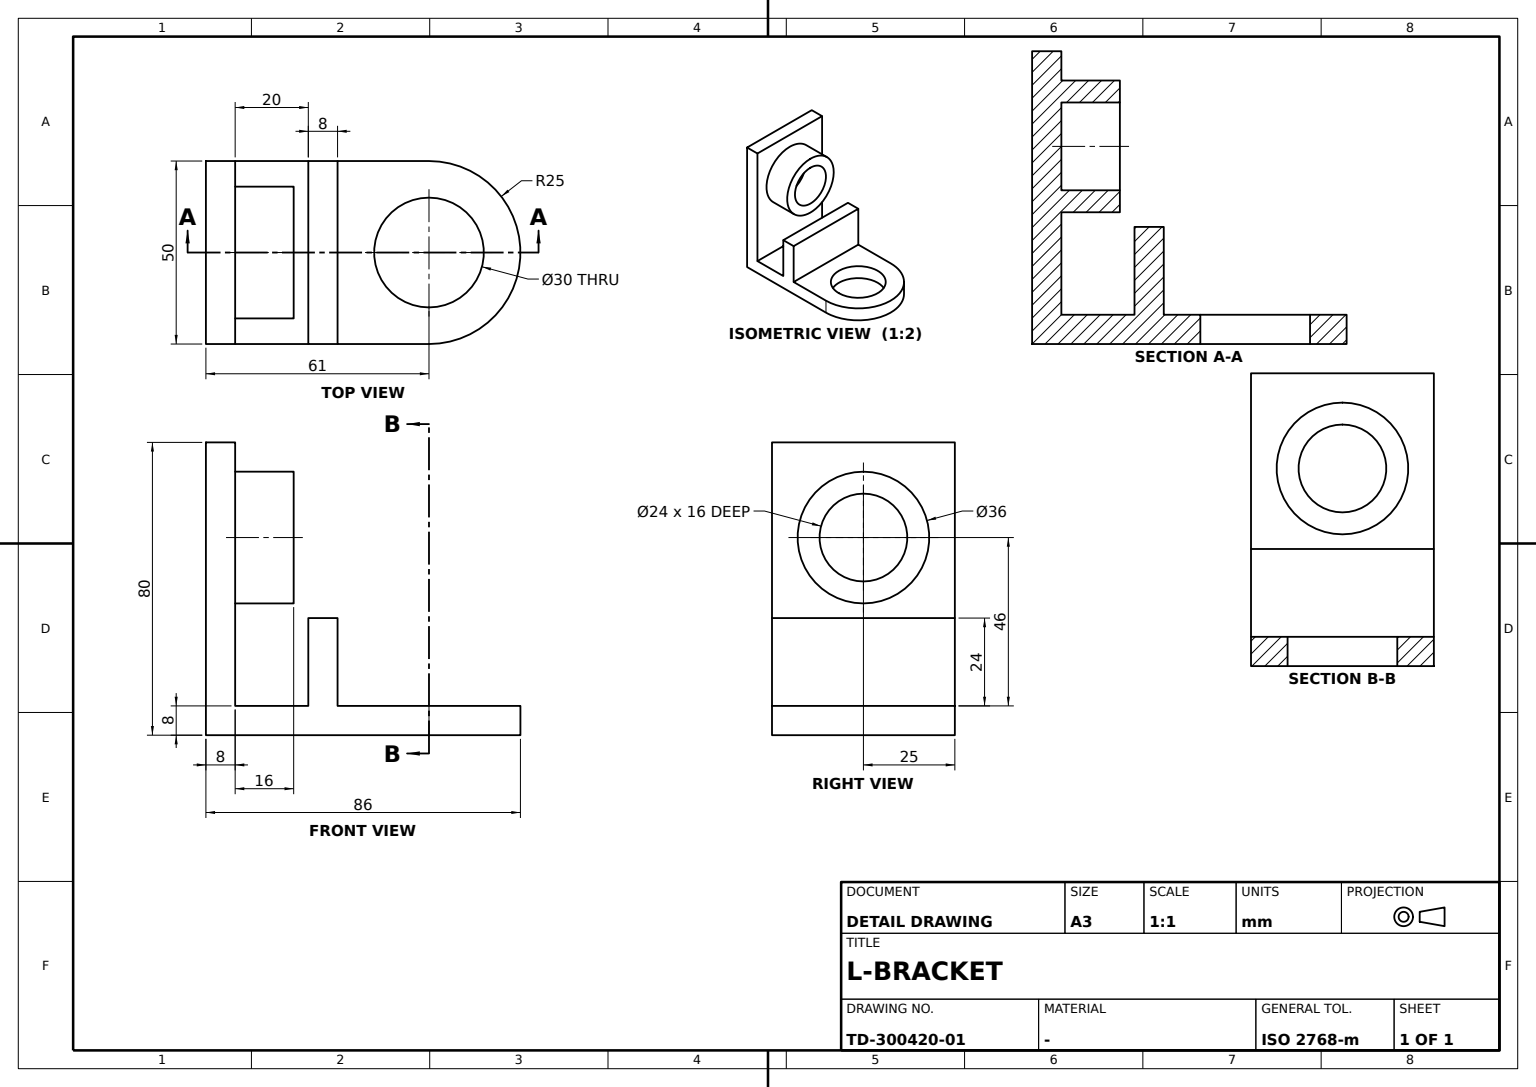
ISO-10303-21;
HEADER;
FILE_DESCRIPTION((''),'2;1');
FILE_NAME('','',(''),(''),'','','');
FILE_SCHEMA(('AUTOMOTIVE_DESIGN'));
ENDSEC;
DATA;
#1=APPLICATION_CONTEXT('');
#2=PRODUCT_CONTEXT('',#1,'mechanical');
#3=PRODUCT('','','',(#2));
#4=PRODUCT_DEFINITION_FORMATION('','',#3);
#5=PRODUCT_DEFINITION_CONTEXT('',#1,'design');
#6=PRODUCT_DEFINITION('','',#4,#5);
#7=PRODUCT_DEFINITION_SHAPE('','',#6);
#8=(LENGTH_UNIT()NAMED_UNIT(*)SI_UNIT(.MILLI.,.METRE.));
#9=(NAMED_UNIT(*)PLANE_ANGLE_UNIT()SI_UNIT($,.RADIAN.));
#10=(NAMED_UNIT(*)SI_UNIT($,.STERADIAN.)SOLID_ANGLE_UNIT());
#11=UNCERTAINTY_MEASURE_WITH_UNIT(LENGTH_MEASURE(0.005),#8,'distance_accuracy_value','');
#12=(GEOMETRIC_REPRESENTATION_CONTEXT(3)GLOBAL_UNCERTAINTY_ASSIGNED_CONTEXT((#11))GLOBAL_UNIT_ASSIGNED_CONTEXT((#8,#9,#10))REPRESENTATION_CONTEXT('',''));
#13=CARTESIAN_POINT('',(25.,8.,80.));
#14=VERTEX_POINT('',#13);
#15=CARTESIAN_POINT('',(25.,0.,80.));
#16=VERTEX_POINT('',#15);
#17=DIRECTION('',(0.,-1.,0.));
#18=VECTOR('',#17,1000.);
#19=LINE('',#15,#18);
#20=EDGE_CURVE('',#14,#16,#19,.T.);
#21=ORIENTED_EDGE('',*,*,#20,.T.);
#22=CARTESIAN_POINT('',(25.,0.,0.));
#23=VERTEX_POINT('',#22);
#24=DIRECTION('',(0.,0.,-1.));
#25=VECTOR('',#24,1000.);
#26=LINE('',#22,#25);
#27=EDGE_CURVE('',#16,#23,#26,.T.);
#28=ORIENTED_EDGE('',*,*,#27,.T.);
#29=CARTESIAN_POINT('',(25.,61.,0.));
#30=VERTEX_POINT('',#29);
#31=DIRECTION('',(0.,1.,0.));
#32=VECTOR('',#31,1000.);
#33=LINE('',#22,#32);
#34=EDGE_CURVE('',#23,#30,#33,.T.);
#35=ORIENTED_EDGE('',*,*,#34,.T.);
#36=CARTESIAN_POINT('',(25.,61.,8.));
#37=VERTEX_POINT('',#36);
#38=CARTESIAN_POINT('',(25.,61.,4.));
#39=DIRECTION('',(0.,0.,1.));
#40=VECTOR('',#39,1000.);
#41=LINE('',#38,#40);
#42=EDGE_CURVE('',#30,#37,#41,.T.);
#43=ORIENTED_EDGE('',*,*,#42,.T.);
#44=CARTESIAN_POINT('',(25.,36.,8.));
#45=VERTEX_POINT('',#44);
#46=CARTESIAN_POINT('',(25.,28.,8.));
#47=LINE('',#46,#32);
#48=EDGE_CURVE('',#45,#37,#47,.T.);
#49=ORIENTED_EDGE('',*,*,#48,.F.);
#50=CARTESIAN_POINT('',(25.,36.,32.));
#51=VERTEX_POINT('',#50);
#52=CARTESIAN_POINT('',(25.,36.,0.));
#53=LINE('',#52,#40);
#54=EDGE_CURVE('',#45,#51,#53,.T.);
#55=ORIENTED_EDGE('',*,*,#54,.T.);
#56=CARTESIAN_POINT('',(25.,28.,32.));
#57=VERTEX_POINT('',#56);
#58=CARTESIAN_POINT('',(25.,0.,32.));
#59=LINE('',#58,#32);
#60=EDGE_CURVE('',#57,#51,#59,.T.);
#61=ORIENTED_EDGE('',*,*,#60,.F.);
#62=VERTEX_POINT('',#46);
#63=CARTESIAN_POINT('',(25.,28.,0.));
#64=LINE('',#63,#25);
#65=EDGE_CURVE('',#57,#62,#64,.T.);
#66=ORIENTED_EDGE('',*,*,#65,.T.);
#67=CARTESIAN_POINT('',(25.,8.,8.));
#68=VERTEX_POINT('',#67);
#69=CARTESIAN_POINT('',(25.,0.,8.));
#70=LINE('',#69,#18);
#71=EDGE_CURVE('',#62,#68,#70,.T.);
#72=ORIENTED_EDGE('',*,*,#71,.T.);
#73=CARTESIAN_POINT('',(25.,8.,0.));
#74=LINE('',#73,#40);
#75=EDGE_CURVE('',#68,#14,#74,.T.);
#76=ORIENTED_EDGE('',*,*,#75,.T.);
#77=EDGE_LOOP('',(#21,#28,#35,#43,#49,#55,#61,#66,#72,#76));
#78=FACE_BOUND('',#77,.T.);
#79=DIRECTION('',(1.,0.,0.));
#80=AXIS2_PLACEMENT_3D('',#22,#79,#31);
#81=PLANE('',#80);
#82=ADVANCED_FACE('',(#78),#81,.T.);
#83=CARTESIAN_POINT('',(0.,8.,72.));
#84=VERTEX_POINT('',#83);
#85=CARTESIAN_POINT('',(0.,8.,54.));
#86=AXIS2_PLACEMENT_3D('',#85,#31,#39);
#87=CIRCLE('',#86,18.);
#88=EDGE_CURVE('',#84,#84,#87,.T.);
#89=ORIENTED_EDGE('',*,*,#88,.F.);
#90=EDGE_LOOP('',(#89));
#91=FACE_BOUND('',#90,.T.);
#92=CARTESIAN_POINT('',(-25.,8.,8.));
#93=VERTEX_POINT('',#92);
#94=CARTESIAN_POINT('',(-25.,8.,80.));
#95=VERTEX_POINT('',#94);
#96=CARTESIAN_POINT('',(-25.,8.,0.));
#97=LINE('',#96,#40);
#98=EDGE_CURVE('',#93,#95,#97,.T.);
#99=ORIENTED_EDGE('',*,*,#98,.T.);
#100=CARTESIAN_POINT('',(0.,8.,80.));
#101=VECTOR('',#79,1000.);
#102=LINE('',#100,#101);
#103=EDGE_CURVE('',#95,#14,#102,.T.);
#104=ORIENTED_EDGE('',*,*,#103,.T.);
#105=ORIENTED_EDGE('',*,*,#75,.F.);
#106=CARTESIAN_POINT('',(0.,8.,8.));
#107=LINE('',#106,#101);
#108=EDGE_CURVE('',#93,#68,#107,.T.);
#109=ORIENTED_EDGE('',*,*,#108,.F.);
#110=EDGE_LOOP('',(#99,#104,#105,#109));
#111=FACE_BOUND('',#110,.T.);
#112=AXIS2_PLACEMENT_3D('',#106,#31,#39);
#113=PLANE('',#112);
#114=ADVANCED_FACE('',(#91,#111),#113,.T.);
#115=CARTESIAN_POINT('',(-25.,28.,8.));
#116=VERTEX_POINT('',#115);
#117=CARTESIAN_POINT('',(0.,28.,8.));
#118=LINE('',#117,#101);
#119=EDGE_CURVE('',#116,#62,#118,.T.);
#120=ORIENTED_EDGE('',*,*,#119,.F.);
#121=CARTESIAN_POINT('',(-25.,0.,8.));
#122=LINE('',#121,#18);
#123=EDGE_CURVE('',#116,#93,#122,.T.);
#124=ORIENTED_EDGE('',*,*,#123,.T.);
#125=ORIENTED_EDGE('',*,*,#108,.T.);
#126=ORIENTED_EDGE('',*,*,#71,.F.);
#127=EDGE_LOOP('',(#120,#124,#125,#126));
#128=FACE_BOUND('',#127,.T.);
#129=AXIS2_PLACEMENT_3D('',#117,#39,#17);
#130=PLANE('',#129);
#131=ADVANCED_FACE('',(#128),#130,.T.);
#132=CARTESIAN_POINT('',(0.,8.,66.));
#133=VERTEX_POINT('',#132);
#134=CIRCLE('',#86,12.);
#135=EDGE_CURVE('',#133,#133,#134,.T.);
#136=ORIENTED_EDGE('',*,*,#135,.T.);
#137=EDGE_LOOP('',(#136));
#138=FACE_BOUND('',#137,.T.);
#139=ADVANCED_FACE('',(#138),#113,.T.);
#140=CARTESIAN_POINT('',(-25.,36.,32.));
#141=VERTEX_POINT('',#140);
#142=CARTESIAN_POINT('',(0.,36.,32.));
#143=LINE('',#142,#101);
#144=EDGE_CURVE('',#141,#51,#143,.T.);
#145=ORIENTED_EDGE('',*,*,#144,.T.);
#146=ORIENTED_EDGE('',*,*,#54,.F.);
#147=CARTESIAN_POINT('',(-25.,36.,8.));
#148=VERTEX_POINT('',#147);
#149=CARTESIAN_POINT('',(0.,36.,8.));
#150=DIRECTION('',(-1.,0.,0.));
#151=VECTOR('',#150,1000.);
#152=LINE('',#149,#151);
#153=EDGE_CURVE('',#45,#148,#152,.T.);
#154=ORIENTED_EDGE('',*,*,#153,.T.);
#155=CARTESIAN_POINT('',(-25.,36.,0.));
#156=LINE('',#155,#40);
#157=EDGE_CURVE('',#148,#141,#156,.T.);
#158=ORIENTED_EDGE('',*,*,#157,.T.);
#159=EDGE_LOOP('',(#145,#146,#154,#158));
#160=FACE_BOUND('',#159,.T.);
#161=CARTESIAN_POINT('',(0.,36.,0.));
#162=AXIS2_PLACEMENT_3D('',#161,#31,#39);
#163=PLANE('',#162);
#164=ADVANCED_FACE('',(#160),#163,.T.);
#165=CARTESIAN_POINT('',(0.,24.,72.));
#166=VERTEX_POINT('',#165);
#167=CARTESIAN_POINT('',(0.,24.,54.));
#168=AXIS2_PLACEMENT_3D('',#167,#31,#39);
#169=CIRCLE('',#168,18.);
#170=EDGE_CURVE('',#166,#166,#169,.T.);
#171=ORIENTED_EDGE('',*,*,#170,.F.);
#172=EDGE_LOOP('',(#171));
#173=FACE_BOUND('',#172,.T.);
#174=ORIENTED_EDGE('',*,*,#88,.T.);
#175=EDGE_LOOP('',(#174));
#176=FACE_BOUND('',#175,.T.);
#177=CARTESIAN_POINT('',(0.,12.,54.));
#178=AXIS2_PLACEMENT_3D('',#177,#31,#150);
#179=CYLINDRICAL_SURFACE('',#178,18.);
#180=ADVANCED_FACE('',(#173,#176),#179,.T.);
#181=CARTESIAN_POINT('',(-25.,61.,8.));
#182=VERTEX_POINT('',#181);
#183=EDGE_CURVE('',#182,#148,#122,.T.);
#184=ORIENTED_EDGE('',*,*,#183,.F.);
#185=CARTESIAN_POINT('',(-25.,61.,0.));
#186=VERTEX_POINT('',#185);
#187=CARTESIAN_POINT('',(-25.,61.,4.));
#188=LINE('',#187,#40);
#189=EDGE_CURVE('',#186,#182,#188,.T.);
#190=ORIENTED_EDGE('',*,*,#189,.F.);
#191=CARTESIAN_POINT('',(-25.,0.,0.));
#192=VERTEX_POINT('',#191);
#193=LINE('',#191,#32);
#194=EDGE_CURVE('',#192,#186,#193,.T.);
#195=ORIENTED_EDGE('',*,*,#194,.F.);
#196=CARTESIAN_POINT('',(-25.,0.,80.));
#197=VERTEX_POINT('',#196);
#198=LINE('',#191,#25);
#199=EDGE_CURVE('',#197,#192,#198,.T.);
#200=ORIENTED_EDGE('',*,*,#199,.F.);
#201=LINE('',#196,#18);
#202=EDGE_CURVE('',#95,#197,#201,.T.);
#203=ORIENTED_EDGE('',*,*,#202,.F.);
#204=ORIENTED_EDGE('',*,*,#98,.F.);
#205=ORIENTED_EDGE('',*,*,#123,.F.);
#206=CARTESIAN_POINT('',(-25.,28.,32.));
#207=VERTEX_POINT('',#206);
#208=CARTESIAN_POINT('',(-25.,28.,0.));
#209=LINE('',#208,#25);
#210=EDGE_CURVE('',#207,#116,#209,.T.);
#211=ORIENTED_EDGE('',*,*,#210,.F.);
#212=CARTESIAN_POINT('',(-25.,0.,32.));
#213=LINE('',#212,#32);
#214=EDGE_CURVE('',#207,#141,#213,.T.);
#215=ORIENTED_EDGE('',*,*,#214,.T.);
#216=ORIENTED_EDGE('',*,*,#157,.F.);
#217=EDGE_LOOP('',(#184,#190,#195,#200,#203,#204,#205,#211,#215,#216));
#218=FACE_BOUND('',#217,.T.);
#219=AXIS2_PLACEMENT_3D('',#191,#79,#31);
#220=PLANE('',#219);
#221=ADVANCED_FACE('',(#218),#220,.F.);
#222=CARTESIAN_POINT('',(15.,61.,8.));
#223=VERTEX_POINT('',#222);
#224=CARTESIAN_POINT('',(0.,61.,8.));
#225=AXIS2_PLACEMENT_3D('',#224,#39,#79);
#226=CIRCLE('',#225,15.);
#227=EDGE_CURVE('',#223,#223,#226,.T.);
#228=ORIENTED_EDGE('',*,*,#227,.F.);
#229=EDGE_LOOP('',(#228));
#230=FACE_BOUND('',#229,.T.);
#231=ORIENTED_EDGE('',*,*,#153,.F.);
#232=ORIENTED_EDGE('',*,*,#48,.T.);
#233=CIRCLE('',#225,25.);
#234=EDGE_CURVE('',#37,#182,#233,.T.);
#235=ORIENTED_EDGE('',*,*,#234,.T.);
#236=ORIENTED_EDGE('',*,*,#183,.T.);
#237=EDGE_LOOP('',(#231,#232,#235,#236));
#238=FACE_BOUND('',#237,.T.);
#239=ADVANCED_FACE('',(#230,#238),#130,.T.);
#240=CARTESIAN_POINT('',(0.,0.,80.));
#241=LINE('',#240,#101);
#242=EDGE_CURVE('',#197,#16,#241,.T.);
#243=ORIENTED_EDGE('',*,*,#242,.T.);
#244=ORIENTED_EDGE('',*,*,#20,.F.);
#245=ORIENTED_EDGE('',*,*,#103,.F.);
#246=ORIENTED_EDGE('',*,*,#202,.T.);
#247=EDGE_LOOP('',(#243,#244,#245,#246));
#248=FACE_BOUND('',#247,.T.);
#249=AXIS2_PLACEMENT_3D('',#100,#39,#17);
#250=PLANE('',#249);
#251=ADVANCED_FACE('',(#248),#250,.T.);
#252=CARTESIAN_POINT('',(0.,24.,66.));
#253=VERTEX_POINT('',#252);
#254=CIRCLE('',#168,12.);
#255=EDGE_CURVE('',#253,#253,#254,.T.);
#256=ORIENTED_EDGE('',*,*,#255,.T.);
#257=EDGE_LOOP('',(#256));
#258=FACE_BOUND('',#257,.T.);
#259=ORIENTED_EDGE('',*,*,#135,.F.);
#260=EDGE_LOOP('',(#259));
#261=FACE_BOUND('',#260,.T.);
#262=CYLINDRICAL_SURFACE('',#178,12.);
#263=ADVANCED_FACE('',(#258,#261),#262,.F.);
#264=CARTESIAN_POINT('',(0.,61.,0.));
#265=AXIS2_PLACEMENT_3D('',#264,#24,#150);
#266=CIRCLE('',#265,25.);
#267=EDGE_CURVE('',#30,#186,#266,.F.);
#268=ORIENTED_EDGE('',*,*,#267,.T.);
#269=ORIENTED_EDGE('',*,*,#189,.T.);
#270=ORIENTED_EDGE('',*,*,#234,.F.);
#271=ORIENTED_EDGE('',*,*,#42,.F.);
#272=EDGE_LOOP('',(#268,#269,#270,#271));
#273=FACE_BOUND('',#272,.T.);
#274=CARTESIAN_POINT('',(0.,61.,4.));
#275=AXIS2_PLACEMENT_3D('',#274,#39,#79);
#276=CYLINDRICAL_SURFACE('',#275,25.);
#277=ADVANCED_FACE('',(#273),#276,.T.);
#278=ORIENTED_EDGE('',*,*,#34,.F.);
#279=CARTESIAN_POINT('',(0.,0.,0.));
#280=LINE('',#279,#101);
#281=EDGE_CURVE('',#192,#23,#280,.T.);
#282=ORIENTED_EDGE('',*,*,#281,.F.);
#283=ORIENTED_EDGE('',*,*,#194,.T.);
#284=ORIENTED_EDGE('',*,*,#267,.F.);
#285=EDGE_LOOP('',(#278,#282,#283,#284));
#286=FACE_BOUND('',#285,.T.);
#287=CARTESIAN_POINT('',(-15.,61.,0.));
#288=VERTEX_POINT('',#287);
#289=CIRCLE('',#265,15.);
#290=EDGE_CURVE('',#288,#288,#289,.F.);
#291=ORIENTED_EDGE('',*,*,#290,.T.);
#292=EDGE_LOOP('',(#291));
#293=FACE_BOUND('',#292,.T.);
#294=AXIS2_PLACEMENT_3D('',#279,#24,#31);
#295=PLANE('',#294);
#296=ADVANCED_FACE('',(#286,#293),#295,.T.);
#297=ORIENTED_EDGE('',*,*,#255,.F.);
#298=EDGE_LOOP('',(#297));
#299=FACE_BOUND('',#298,.T.);
#300=ORIENTED_EDGE('',*,*,#170,.T.);
#301=EDGE_LOOP('',(#300));
#302=FACE_BOUND('',#301,.T.);
#303=CARTESIAN_POINT('',(0.,24.,0.));
#304=AXIS2_PLACEMENT_3D('',#303,#31,#150);
#305=PLANE('',#304);
#306=ADVANCED_FACE('',(#299,#302),#305,.T.);
#307=ORIENTED_EDGE('',*,*,#27,.F.);
#308=ORIENTED_EDGE('',*,*,#242,.F.);
#309=ORIENTED_EDGE('',*,*,#199,.T.);
#310=ORIENTED_EDGE('',*,*,#281,.T.);
#311=EDGE_LOOP('',(#307,#308,#309,#310));
#312=FACE_BOUND('',#311,.T.);
#313=AXIS2_PLACEMENT_3D('',#240,#17,#24);
#314=PLANE('',#313);
#315=ADVANCED_FACE('',(#312),#314,.T.);
#316=ORIENTED_EDGE('',*,*,#119,.T.);
#317=ORIENTED_EDGE('',*,*,#65,.F.);
#318=CARTESIAN_POINT('',(0.,28.,32.));
#319=LINE('',#318,#101);
#320=EDGE_CURVE('',#207,#57,#319,.T.);
#321=ORIENTED_EDGE('',*,*,#320,.F.);
#322=ORIENTED_EDGE('',*,*,#210,.T.);
#323=EDGE_LOOP('',(#316,#317,#321,#322));
#324=FACE_BOUND('',#323,.T.);
#325=AXIS2_PLACEMENT_3D('',#318,#17,#24);
#326=PLANE('',#325);
#327=ADVANCED_FACE('',(#324),#326,.T.);
#328=ORIENTED_EDGE('',*,*,#60,.T.);
#329=ORIENTED_EDGE('',*,*,#144,.F.);
#330=ORIENTED_EDGE('',*,*,#214,.F.);
#331=ORIENTED_EDGE('',*,*,#320,.T.);
#332=EDGE_LOOP('',(#328,#329,#330,#331));
#333=FACE_BOUND('',#332,.T.);
#334=AXIS2_PLACEMENT_3D('',#318,#24,#31);
#335=PLANE('',#334);
#336=ADVANCED_FACE('',(#333),#335,.F.);
#337=ORIENTED_EDGE('',*,*,#290,.F.);
#338=EDGE_LOOP('',(#337));
#339=FACE_BOUND('',#338,.T.);
#340=ORIENTED_EDGE('',*,*,#227,.T.);
#341=EDGE_LOOP('',(#340));
#342=FACE_BOUND('',#341,.T.);
#343=CYLINDRICAL_SURFACE('',#275,15.);
#344=ADVANCED_FACE('',(#339,#342),#343,.F.);
#345=CLOSED_SHELL('',(#82,#114,#131,#139,#164,#180,#221,#239,#251,#263,#277,#296,#306,#315,#327,#336,#344));
#346=MANIFOLD_SOLID_BREP('',#345);
#347=ADVANCED_BREP_SHAPE_REPRESENTATION('',(#346),#12);
#348=SHAPE_DEFINITION_REPRESENTATION(#7,#347);
ENDSEC;
END-ISO-10303-21;
